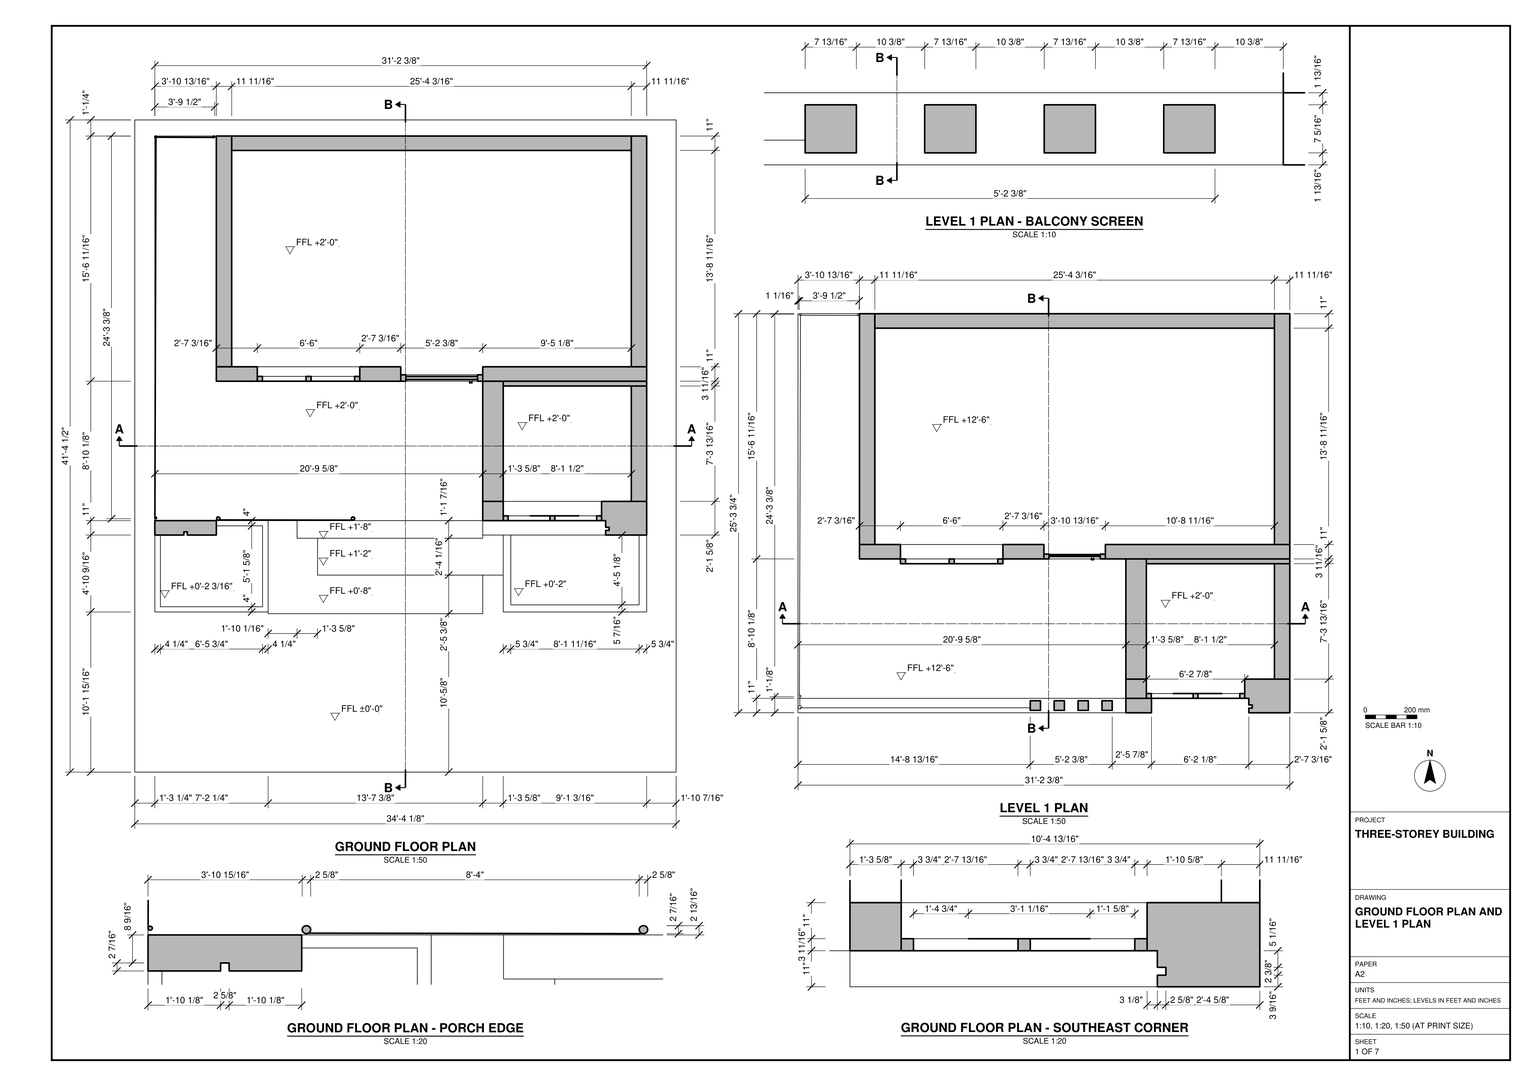
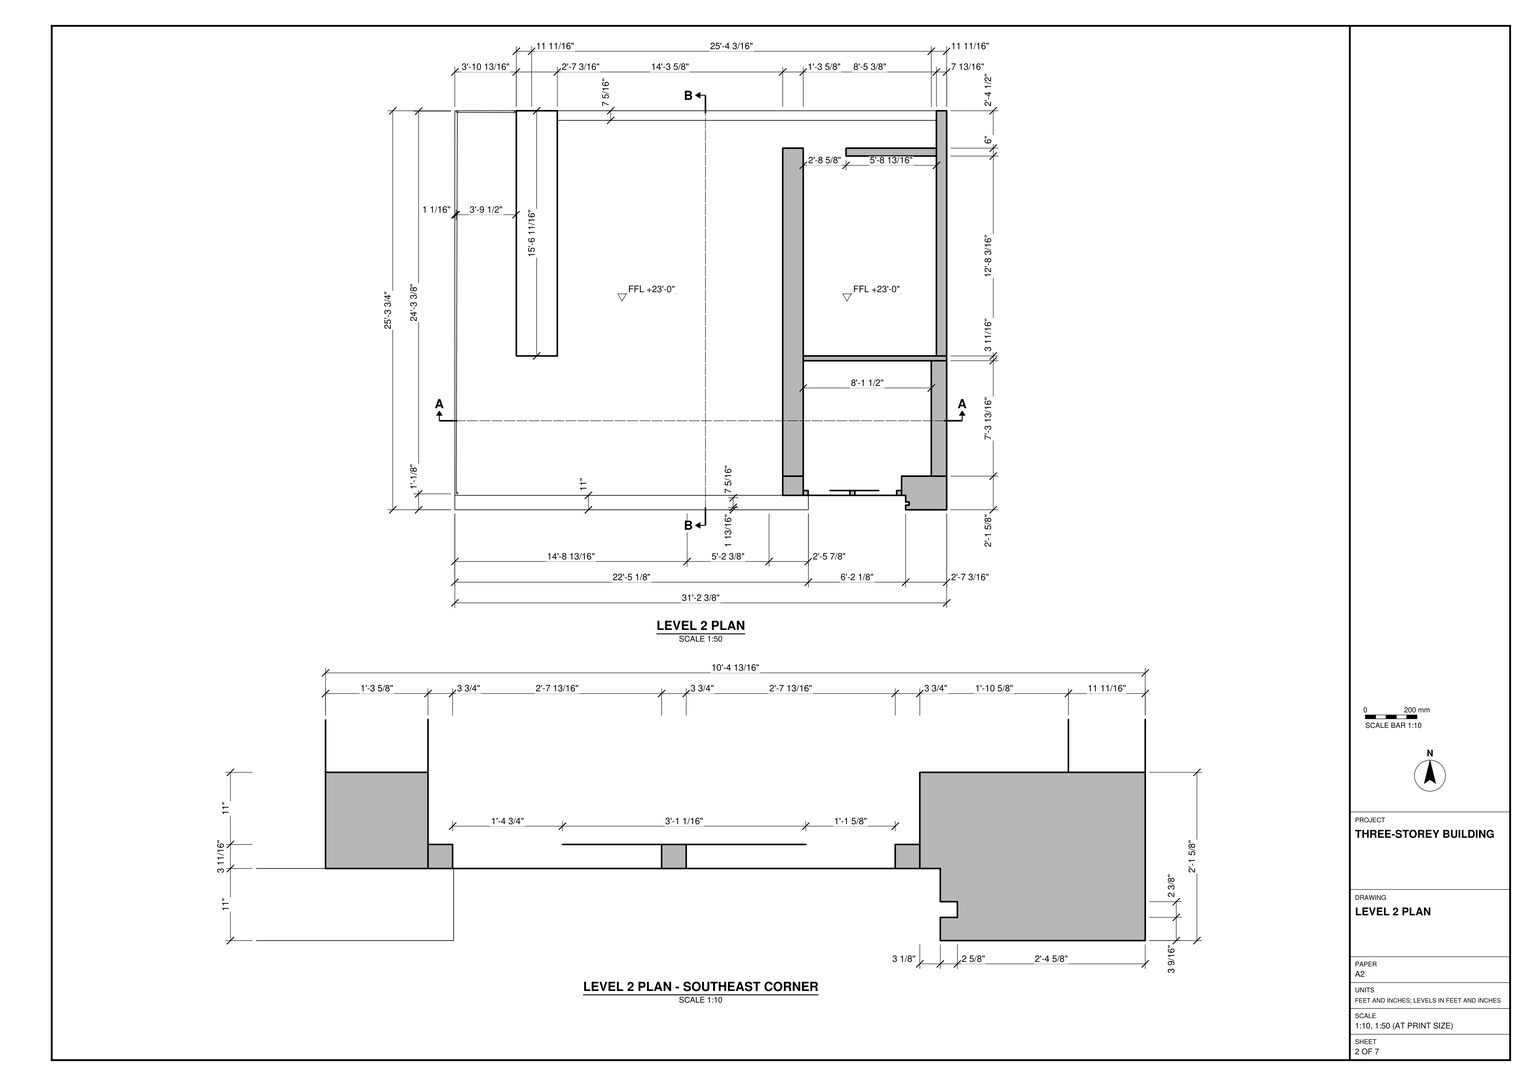
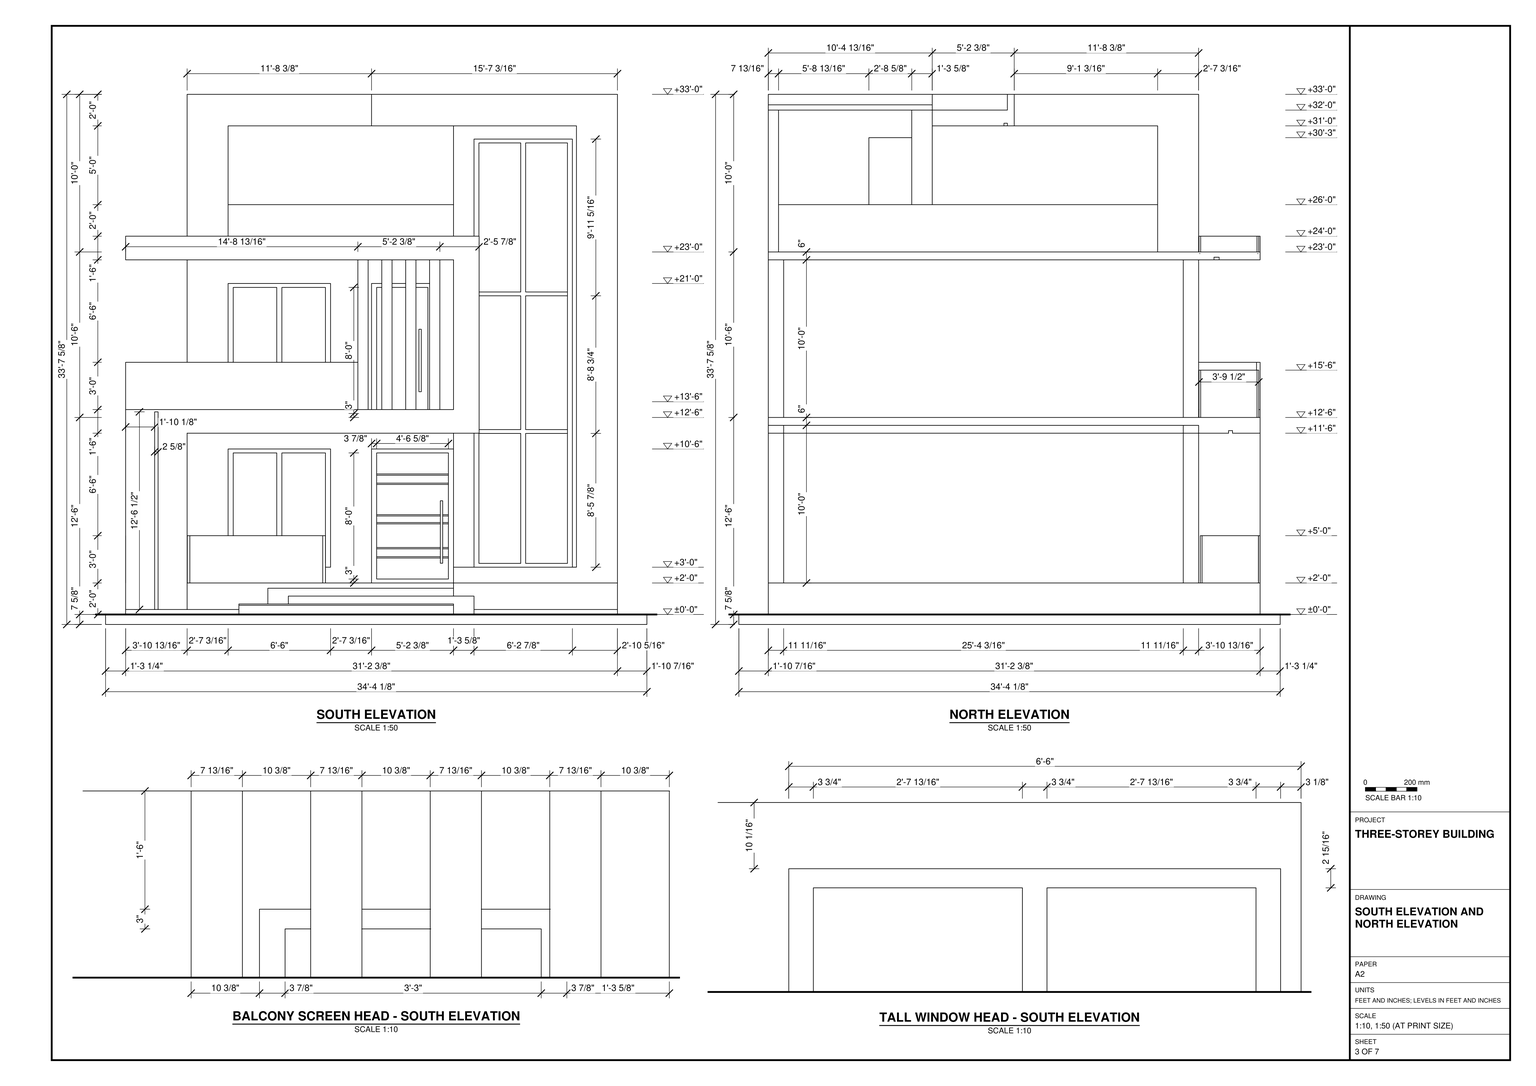
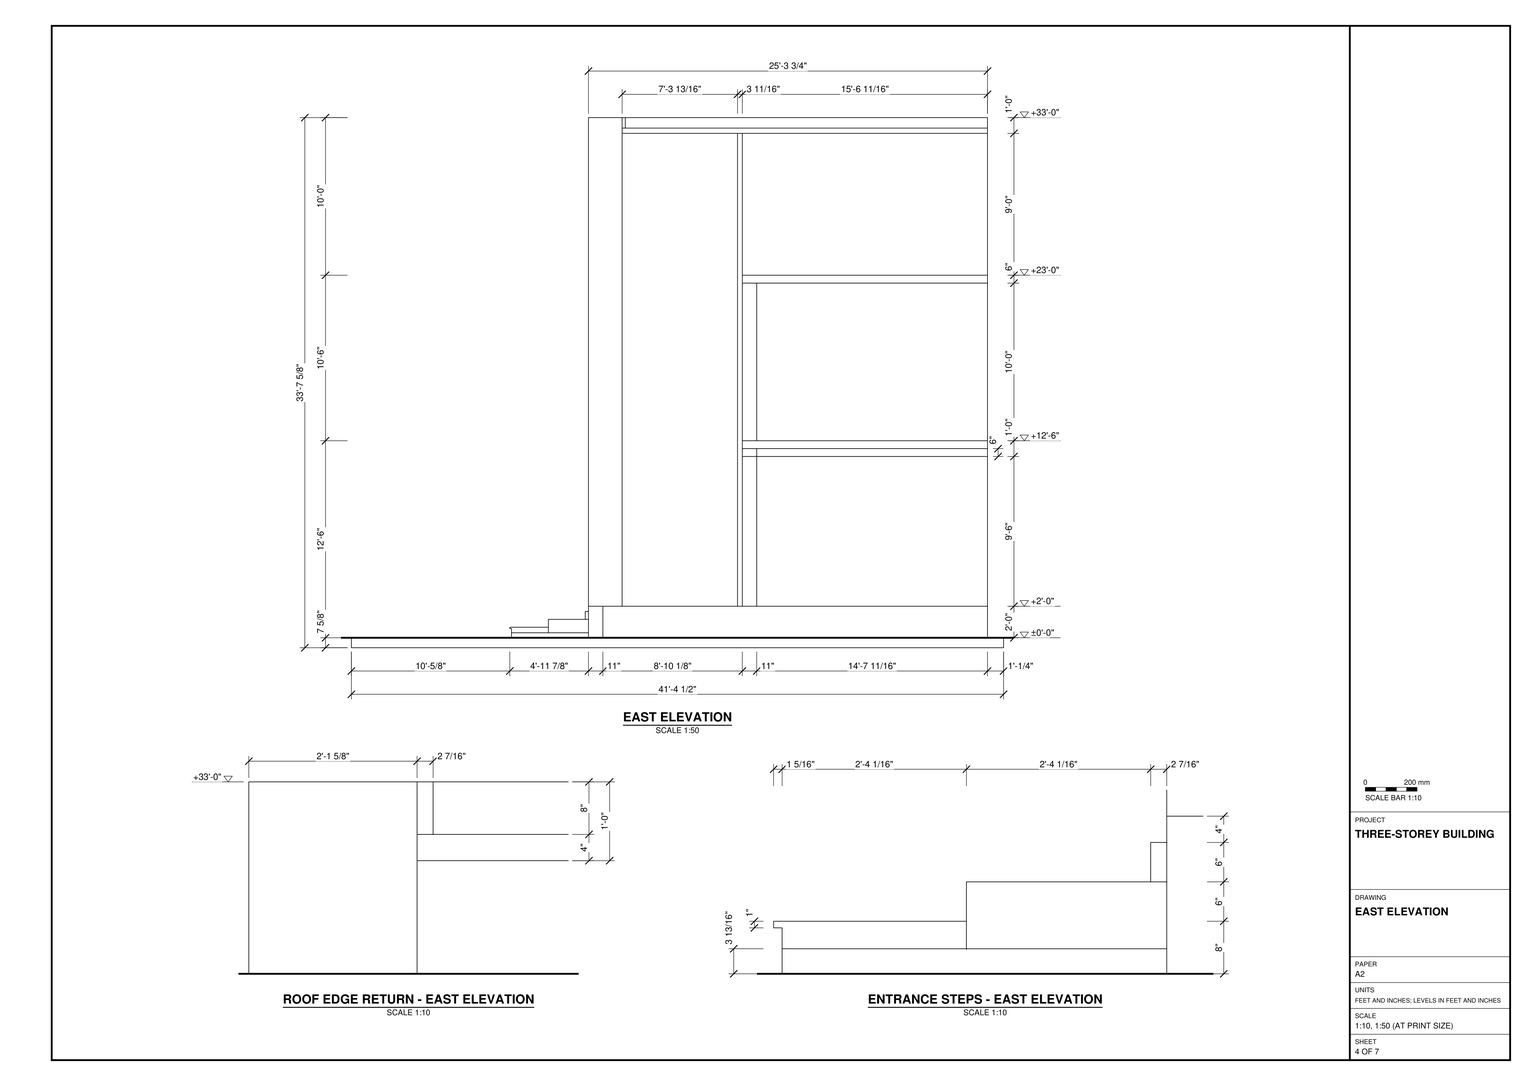
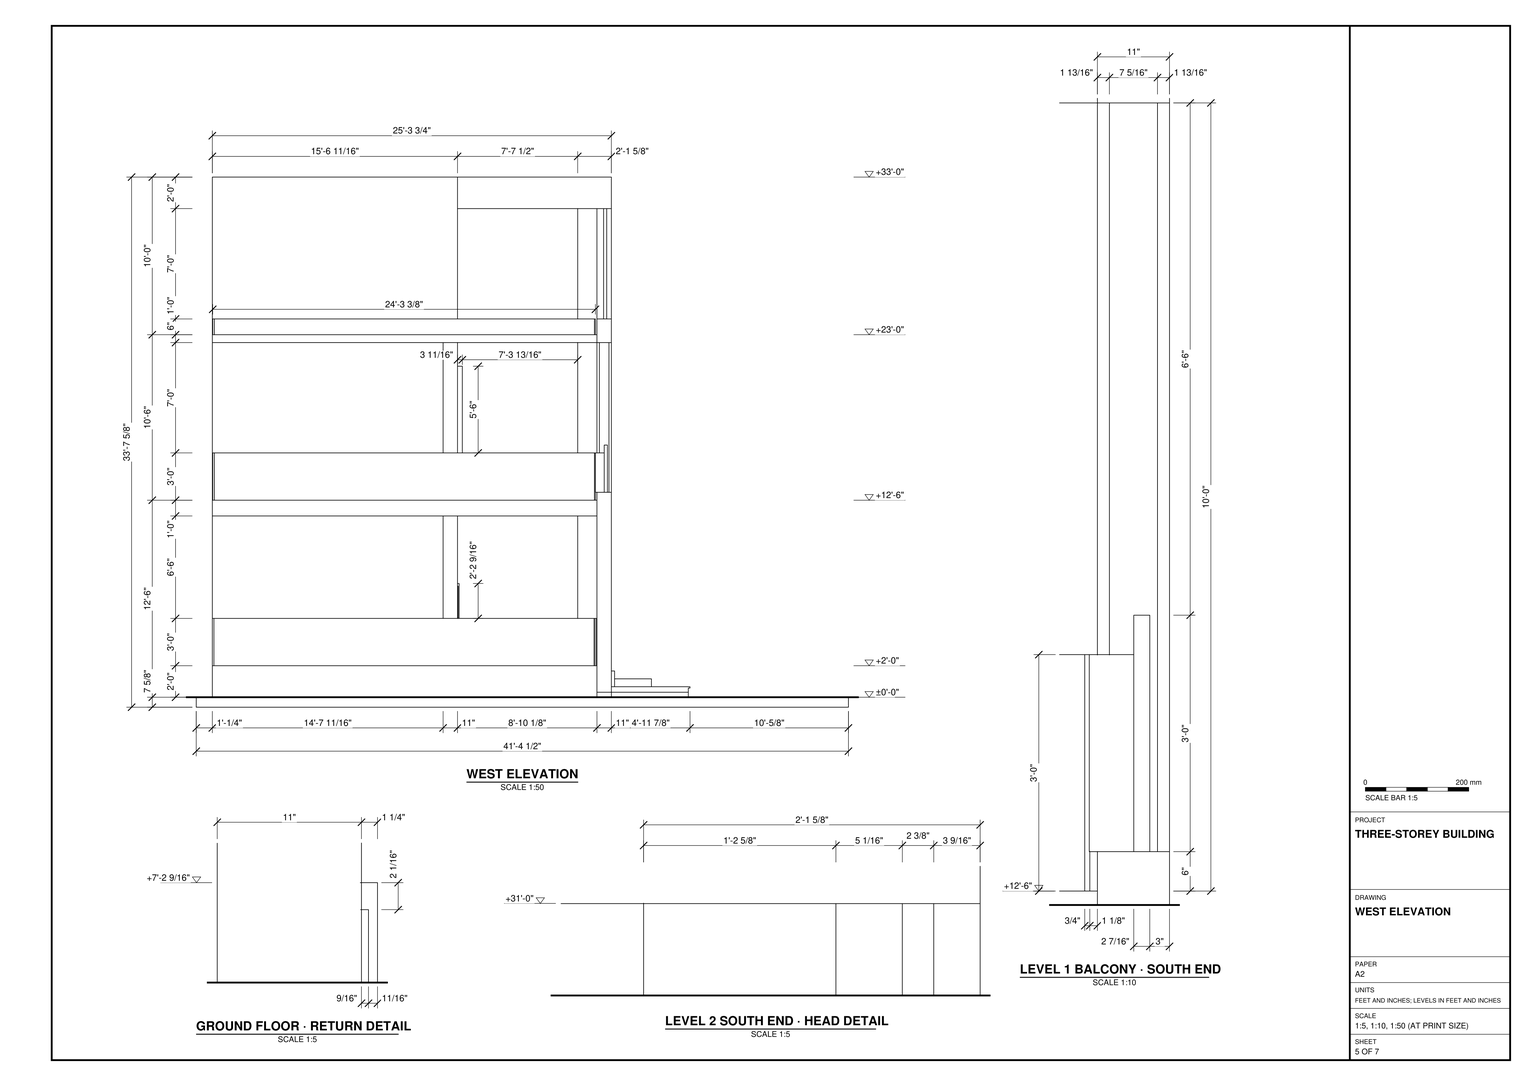
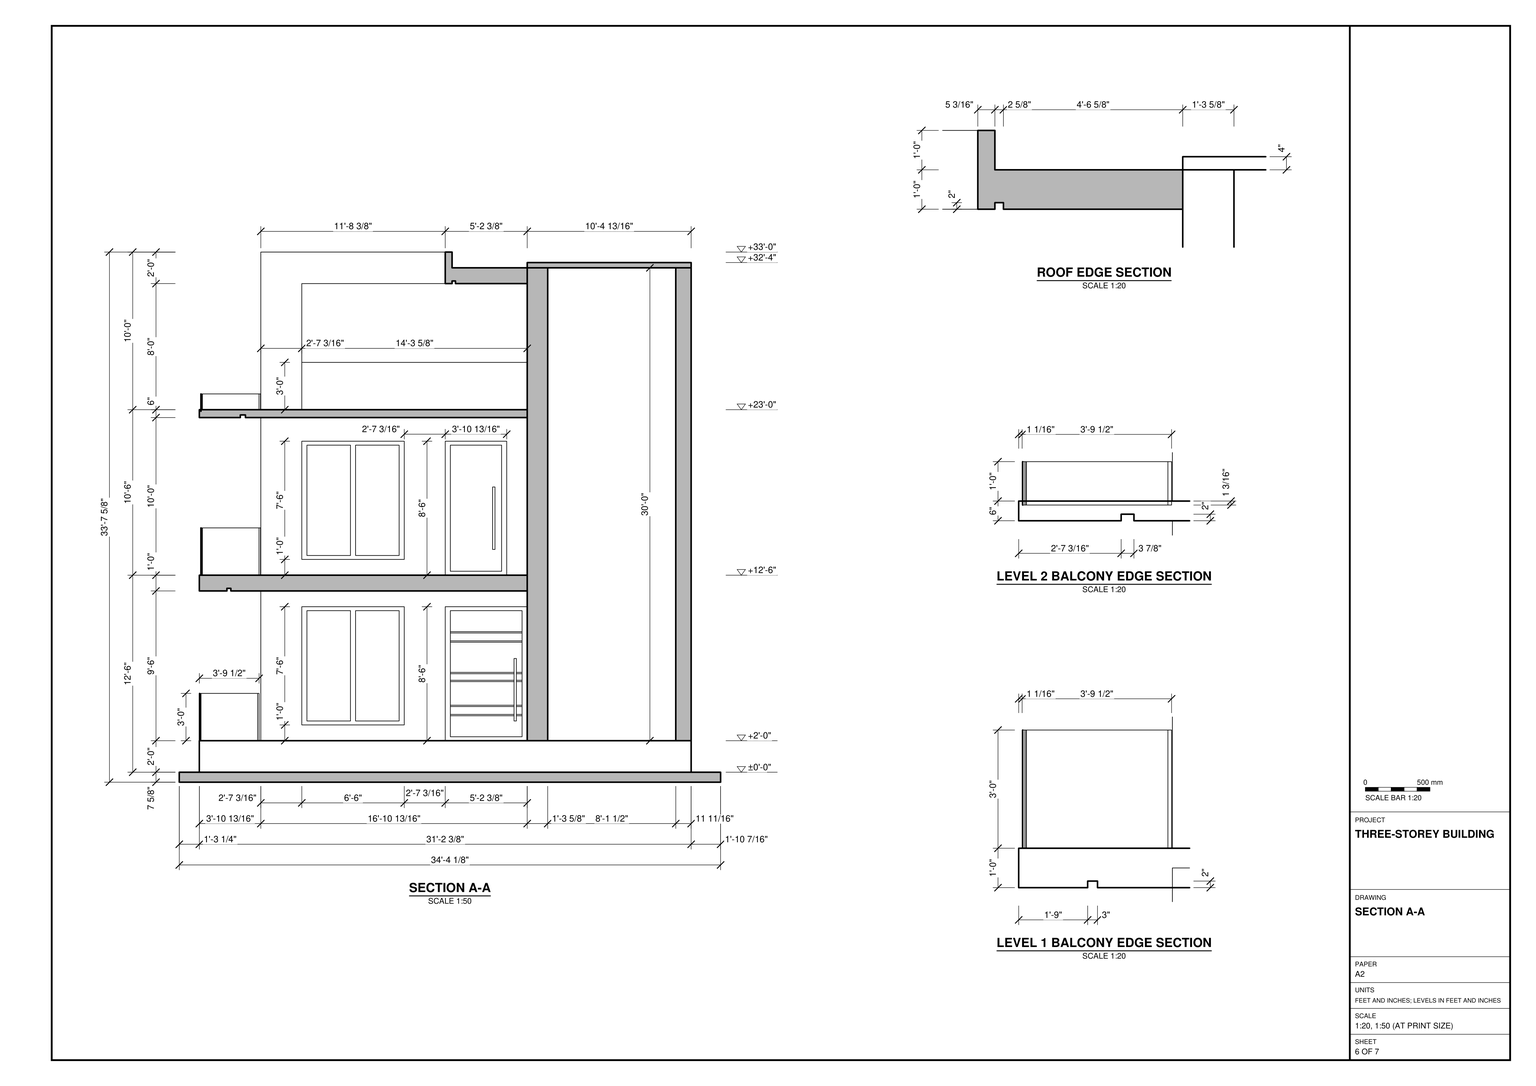
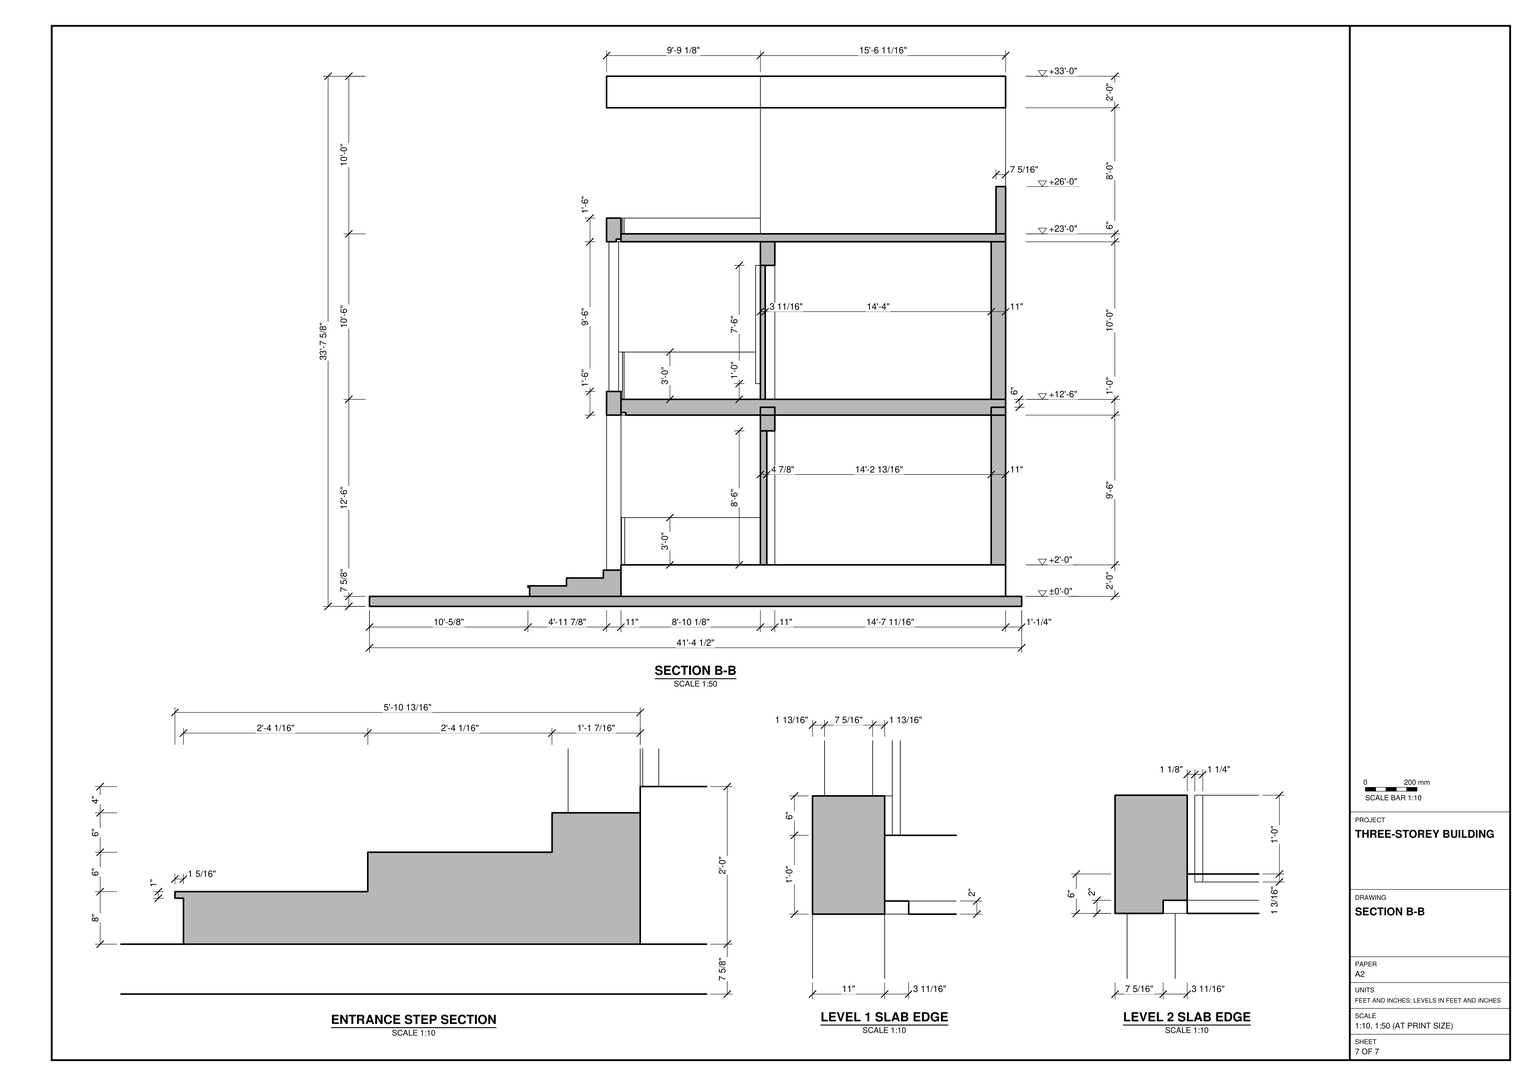
Build the three-storey building shown in task_files/diagram_01.pdf. Work in feet and inches. Including the base slab, the model must measure 34'-4 1/8" east to west, 41'-4 1/2" north to south and 33'-7 5/8" from bottom to top. Use ±0'-0" as the ground datum, +12'-6" for Level 1 and +23'-0" for Level 2. Distinguish the raised entrance floor from the ground datum.

Lay out the broad rear enclosure, the south-facing porch and the narrower southeast bay from the plans. Model the entrance steps, porch edge, walls at their drawn thicknesses, door and window openings, and projecting floor slabs. Align the Level 1 balcony with the porch below. Follow the enlarged details for the spacing of the balcony screen and the subdivisions of the tall southeast window. At Level 2, use the plan and elevations together to distinguish solid wall panels from open areas beneath the roof frame.

Keep walls, slabs, roof elements and each furniture or joinery piece shown in separate groups or components, and use components for repeated parts. Any decor or loose items shown may be represented by suitable library components. Save one SketchUp model as output_files/three_storey_building_with_a_screened_balcony.skp.

# SketchUp Ruby script. Lengths in inches.
U = 1.inch
M = Sketchup.active_model
def pt(a) = Geom::Point3d.new(a.map { |v| v * U })
def face(e, loops, mat)
  f = e.add_face(loops[0].map { |a| pt(a) })
  loops[1..].each { |l| e.add_face(l.map { |a| pt(a) }).erase! }
  f.material = f.back_material = mat if mat
  f
end
# faces: each face lists its corners as indices into pts; further lists are holes
def faces(e, pts, list, mat = nil) = list.each { |f| face(e, (f[0].is_a?(Array) ? f : [f]).map { |l| l.map { |i| pts[i] } }, mat) }
# xy, xz, yz: faces in a plane at the given z, y or x. An outline is a flat list of corners, or four numbers for a rectangle; further outlines are holes
def ring(l) = l.size == 4 ? [[l[0], l[1]], [l[2], l[1]], [l[2], l[3]], [l[0], l[3]]] : l.each_slice(2).to_a
def flat(e, list, mat, &to3) = list.each { |f| face(e, (f[0].is_a?(Array) ? f : [f]).map { |l| ring(l).map { |u, v| to3.(u, v) } }, mat) }
def xy(e, z, list, mat = nil) = flat(e, list, mat) { |x, y| [x, y, z] }
def xz(e, y, list, mat = nil) = flat(e, list, mat) { |x, z| [x, y, z] }
def yz(e, x, list, mat = nil) = flat(e, list, mat) { |y, z| [x, y, z] }
def lines(e, pts, list) = list.each { |a, b| e.add_line(pt(pts[a]), pt(pts[b])) }
# prism: a flat outline (further loops are holes) pulled along v
def prism(e, loops, v, mat = nil)
  f = face(e, loops, mat); d = Geom::Vector3d.new(v.map { |x| x * U })
  f.pushpull(f.normal.samedirection?(d) ? d.length : -d.length)
end
def box(e, o, s, mat = nil) = prism(e, [[o, [o[0] + s[0], o[1], o[2]], [o[0] + s[0], o[1] + s[1], o[2]], [o[0], o[1] + s[1], o[2]]]], [0, 0, s[2]], mat)
def at(x, y, z, deg = 0) = Geom::Transformation.translation(pt([x, y, z])) * Geom::Transformation.rotation(ORIGIN, Z_AXIS, deg.degrees)
def axes(o, x, y, z) = Geom::Transformation.new([*x, 0, *y, 0, *z, 0, *pt(o).to_a, 1])
def part(name) = M.definitions.add(name)
# library, detail: a bought-in or finely detailed component or shape, given as its bounding box
def library(name, o, s) = part(name).tap { |d| box(d.entities, o, s) }
def detail(e, o, s) = box(e.add_group.entities, o, s)
def put(e, d, t, mat = nil) = e.add_instance(d, t).tap { |i| i.material = mat if mat }
def group(e, t, mat = nil) = e.add_group.tap { |g| g.transformation = t; g.material = mat if mat }.entities
root = M.entities
M.materials.add("[Blinds Vertical Pattern]").color = [252, 252, 255]
M.materials.add("[Color G08]").color = [0, 102, 0]
M.materials.add("[Color M00]").color = [255, 255, 255]
M.materials.add("[Color M03]").color = [170, 170, 170]
M.materials.add("[Color M09]").color = [0, 0, 0]
M.materials.add("[Grass Dark Green]").color = [106, 157, 55]
M.materials.add("[Marble Carrara Floor Tile]").color = [204, 208, 219]
M.materials.add("[Marble Carrara Gold Floor Tile]").color = [225, 223, 217]
M.materials.add("[Metal Corrugated Shiny]").color = [193, 193, 193]
M.materials.add("[Metal Seamed]").color = [118, 119, 115]
M.materials.add("[Tile Mosaic Multi]").color = [160, 122, 114]
M.materials.add("[Translucent Glass Gray]").color = [255, 255, 255]
M.materials["[Translucent Glass Gray]"].alpha = 0.5
M.materials.add("[Translucent Glass Tinted]").color = [8, 201, 241]
M.materials["[Translucent Glass Tinted]"].alpha = 0.14
M.materials.add("[Wood Cherry Original]").color = [152, 86, 42]
M.materials.add("[Wood Veneer 02]").color = [190, 128, 91]
c1 = part("Group\#7")
xz(c1.entities,0,[[3,3,28.5,87],[31.5,3,57,87]],"[Translucent Glass Tinted]")
g1 = group(c1.entities,at(0,0,0),"[Color M09]")
prism(g1,[[[0,0,90],[0,0,0],[60,0,0],[60,0,90]],[[28.5,0,87],[28.5,0,3],[3,0,3],[3,0,87]],[[31.5,0,87],[57,0,87],[57,0,3],[31.5,0,3]]],[0,3,0])
c2 = part("Group\#8")
prism(c2.entities,[[[1.375,2,45.51],[1.375,2,47.5625],[1.375,0,47.5625],[1.375,0,0],[1.375,2,0],[1.375,2,1.44],[1.375,0.5625,1.44],[1.375,0.5625,45.51]]],[-1.375,0,0])
c3 = part("Group\#35")
prism(c3.entities,[[[1.26,1.97,0],[1.5,1.87,0],[1.71,1.71,0],[1.87,1.5,0],[1.97,1.26,0],[2,1,0],[1.97,0.74,0],[1.87,0.5,0],[1.71,0.29,0],[1.5,0.13,0],[1.26,0.03,0],[1,0,0],[0.74,0.03,0],[0.5,0.13,0],[0.29,0.29,0],[0.13,0.5,0],[0.03,0.74,0],[0,1,0],[0.03,1.26,0],[0.13,1.5,0],[0.29,1.71,0],[0.5,1.87,0],[0.74,1.97,0],[1,2,0]]],[0,0,36])
c4 = part("Group\#34")
prism(c4.entities,[[[0.5,0,0],[0.37,0.02,0],[0.25,0.07,0],[0.15,0.15,0],[0.07,0.25,0],[0.02,0.37,0],[0,0.5,0],[0.02,0.63,0],[0.07,0.75,0],[0.15,0.85,0],[0.25,0.93,0],[0.37,0.98,0],[0.5,1,0],[0.63,0.98,0],[0.75,0.93,0],[0.85,0.85,0],[0.93,0.75,0],[0.98,0.63,0],[1,0.5,0],[0.98,0.37,0],[0.93,0.25,0],[0.85,0.15,0],[0.75,0.07,0],[0.63,0.02,0]]],[0,0,36])
c5 = part("Group\#44")
p = [[0.82,237.83,36],[0.02,0.63,36],[0.02,0.63,0],[0.82,237.83,0],[44.39,237.96,0],[44.39,237.96,36],
  [1.21,238.0625,36],[1.21,238.0625,0]]
faces(c5.entities,p,[[0,1,2,3],[4,5,6,7]],"[Translucent Glass Gray]")
put(c5.entities,c4,axes([44.2,237.8125,0],[1.3,0,0],[0,1,0],[0,0,1]))
put(c5.entities,c4,axes([0,237.8125,0],[1.3,0,0],[0,1,0],[0,0,1]))
put(c5.entities,c4,axes([0,0,0],[1.3,0,0],[0,1,0],[0,0,1]))
prism(root,[[[313.09,449.78,269.85],[381.88,449.78,269.85],[381.88,449.78,377.85],[280.48,449.78,377.85],[280.48,449.78,356.87],[313.09,449.78,356.87]]],[0,6,0])
xy(root,17.85,[[377.98,206.09,389.68,293.93]])
xy(root,377.85,[[377.98,206.09,389.68,293.93]])
xz(root,206.09,[[377.98,17.85,389.68,377.85]])
xz(root,293.93,[[377.98,17.85,389.68,377.85]])
yz(root,377.98,[[206.09,17.85,293.93,377.85]])
p = [[64.16,191.99,53.85],[165.32,191.83,53.85],[165.32,191.83,17.85],[64.16,191.99,17.85],[16.66,192.6875,179.85],[16.64,185.91,179.85],
  [16.64,185.91,149.85],[16.66,192.6875,149.85],[264.88,137.77,-0.15],[101.5,137.77,-0.15],[264.88,137.77,0.85],[101.5,137.77,0.85]]
faces(root,p,[[0,1,2,3],[4,5,6,7]],"[Translucent Glass Gray]")
lines(root,p,[[8,9],[10,11]])
g2 = group(root,at(62.08,191.45,-6.15),"[Marble Carrara Floor Tile]")
box(g2,[-46.8,0,0],[374.4,292.8,24])
g3 = group(root,at(73.78,297.59,17.85),"[Color M03]")
prism(g3,[[[315.9,10.98,0],[191.1,10.98,0],[191.1,10.98,102],[128.7,10.98,102],[128.7,10.98,0],[-11.7,10.98,0],[-11.7,10.98,120],[315.9,10.98,120]],[[97.5,10.98,12],[97.5,10.98,102],[19.5,10.98,102],[19.5,10.98,12]]],[0,-10.98,0])
g4 = group(root,at(202.48,296.37,17.85))
g5 = group(g4,at(0,2.44,0),"[Wood Cherry Original]")
prism(g5,[[[0,3.66,0],[0,3.66,102],[62.4,3.66,102],[62.4,3.66,0]],[[3.9,3.66,99],[3.9,3.66,3],[58.5,3.66,3],[58.5,3.66,99]]],[0,-4.88,0])
g6 = group(g4,at(3.9,2.44,3),"[Wood Cherry Original]")
xy(g6,0,[[0,0,54.6,2.44]])
xy(g6,16,[[0,0,54.6,0.61]])
xy(g6,17,[[0,0,54.6,0.61]])
xy(g6,23,[[0,0,54.6,0.61]])
xy(g6,24,[[0,0,54.6,0.61]])
xy(g6,42,[[0,0,54.6,0.61]])
xy(g6,43,[[0,0,54.6,0.61]])
xy(g6,48,[[0,0,54.6,0.61]])
xy(g6,49,[[0,0,54.6,0.61]])
xy(g6,72,[[0,0,54.6,0.61]])
xy(g6,73,[[0,0,54.6,0.61]])
xy(g6,79,[[0,0,54.6,0.61]])
xy(g6,80,[[0,0,54.6,0.61]])
xy(g6,96,[[0,0,54.6,2.44]])
xz(g6,0,[[0,0,54.6,16],[0,17,54.6,23],[0,43,54.6,48],[0,49,54.6,72],[0,73,54.6,79],
  [0,80,54.6,96]])
xz(g6,0,[[0,24,54.6,42]],"[Wood Cherry Original]")
xz(g6,0.61,[[0,16,54.6,17],[0,23,54.6,24],[0,42,54.6,43],[0,48,54.6,49],[0,72,54.6,73],
  [0,79,54.6,80]])
xz(g6,2.44,[[0,0,54.6,96]])
yz(g6,0,[[0,0,0,16,0.61,16,0.61,17,0,17,0,23,0.61,23,0.61,24,0,24,0,42,0.61,42,0.61,43,0,43,0,48,0.61,48,0.61,49,0,49,0,72,0.61,72,0.61,73,0,73,0,79,0.61,79,0.61,80,0,80,0,96,2.44,96,2.44,0]])
yz(g6,54.6,[[0,0,2.44,0,2.44,96,0,96,0,80,0.61,80,0.61,79,0,79,0,73,0.61,73,0.61,72,0,72,0,49,0.61,49,0.61,48,0,48,0,43,0.61,43,0.61,42,0,42,0,24,0.61,24,0.61,23,0,23,0,17,0.61,17,0.61,16,0,16]])
put(root,c1,axes([93.28,297.59,29.85],[1.3,0,0],[0,1.22,0],[0,0,1]))
put(root,c2,axes([254.84,296.37,32.88],[1.3,0,0],[0,1.22,0],[0,0,1]),"[Metal Seamed]")
g7 = group(root,at(62.08,308.57,17.85))
box(g7,[0,0,0],[11.7,175.68,120])
g8 = group(root,at(73.78,473.27,17.85))
box(g8,[0,0,0],[304.2,10.98,120])
g9 = group(root,at(377.98,308.57,17.85))
box(g9,[0,0,0],[11.7,175.68,120])
g10 = group(root,at(62.08,297.59,137.85))
xy(g10,-6,[[-46.8,-106.14,-25.8,186.66],[-22.8,-102.48,-22.8,186.66,327.6,186.66,327.6,0,202.8,0,202.8,-102.48]])
xy(g10,-4,[[-25.8,-106.14,202.8,-102.48],[-25.8,-102.48,-22.8,186.66]],"[Color M09]")
xy(g10,6,[[-46.8,-106.14,202.8,-106.14,202.8,0,327.6,0,327.6,186.66,-46.8,186.66]])
xz(g10,-106.14,[[-46.8,-6,-25.8,-6,-25.8,-4,202.8,-4,202.8,6,-46.8,6]])
xz(g10,-102.48,[[-22.8,-6,202.8,-4]],"[Color M09]")
xz(g10,0,[[202.8,-6,327.6,6]])
xz(g10,186.66,[[-46.8,-6,-46.8,6,327.6,6,327.6,-6,-22.8,-6,-22.8,-4,-25.8,-4,-25.8,-6]])
yz(g10,-46.8,[[-106.14,-6,186.66,6]])
yz(g10,-25.8,[[-106.14,-6,-102.48,-4],[-102.48,-6,186.66,-4]],"[Color M09]")
yz(g10,-22.8,[[-102.48,-6,186.66,-4]],"[Color M09]")
yz(g10,202.8,[[-102.48,-6,0,-6,0,6,-106.14,6,-106.14,-4,-102.48,-4]])
yz(g10,327.6,[[0,-6,186.66,6]])
g11 = group(root,at(62.08,297.59,143.85),"[Color M03]")
prism(g11,[[[140.4,10.98,0],[0,10.98,0],[0,10.98,120],[327.6,10.98,120],[327.6,10.98,0],[187.2,10.98,0],[187.2,10.98,102],[140.4,10.98,102]],[[31.2,10.98,102],[31.2,10.98,12],[109.2,10.98,12],[109.2,10.98,102]]],[0,-10.98,0])
g12 = group(root,at(377.98,308.57,143.85))
box(g12,[0,0,0],[11.7,175.68,120])
g13 = group(root,at(73.78,473.27,143.85))
box(g13,[0,0,0],[304.2,10.98,120])
g14 = group(root,at(62.08,308.57,143.85))
box(g14,[0,0,0],[11.7,175.68,120])
put(root,c1,axes([93.28,293.93,155.85],[1.3,0,0],[0,1.22,0],[0,0,1]))
g15 = group(root,at(202.48,297.59,143.85),"[Wood Cherry Original]")
prism(g15,[[[46.8,3.66,0],[0,3.66,0],[0,3.66,102],[46.8,3.66,102]],[[42.9,3.66,99],[3.9,3.66,99],[3.9,3.66,3],[42.9,3.66,3]]],[0,-3.66,0])
g16 = group(root,at(206.38,299.42,146.85),"[Wood Cherry Original]")
box(g16,[0,0,0],[39,1.22,96])
put(root,c2,axes([238.55,296.98,163.44],[1.3,0,0],[0,1.22,0],[0,0,1]),"[Metal Seamed]")
g17 = group(root,at(62.08,297.59,263.85))
xy(g17,0,[[-46.8,-106.14,-15.6,186.66],[-11.7,-106.14,-11.7,186.66,327.6,186.66,327.6,0,202.8,0,202.8,-106.14]])
xy(g17,2,[[-15.6,-106.14,-11.7,186.66]],"[Color M09]")
xy(g17,6,[[-46.8,-106.14,202.8,-106.14,202.8,0,327.6,0,327.6,186.66,-46.8,186.66]])
xz(g17,-106.14,[[-46.8,0,-15.6,0,-15.6,2,-11.7,2,-11.7,0,202.8,0,202.8,6,-46.8,6]],"[Color M09]")
xz(g17,0,[[202.8,0,327.6,6]])
xz(g17,186.66,[[-46.8,0,-46.8,6,327.6,6,327.6,0,-11.7,0,-11.7,2,-15.6,2,-15.6,0]])
yz(g17,-46.8,[[-106.14,0,186.66,6]])
yz(g17,-15.6,[[-106.14,0,186.66,2]],"[Color M09]")
yz(g17,-11.7,[[-106.14,0,186.66,2]],"[Color M09]")
yz(g17,202.8,[[-106.14,0,0,6]])
yz(g17,327.6,[[0,0,186.66,6]])
g18 = group(root,at(264.88,206.09,17.85),"[Color M09]")
xy(g18,0,[[0,0,15.6,91.5]])
xy(g18,252,[[0,91.5,15.6,249.6875]])
xy(g18,360,[[0,0,15.6,249.6875]],"[Color M00]")
xz(g18,0,[[0,0,15.6,360]])
xz(g18,91.5,[[0,0,15.6,252]])
xz(g18,249.6875,[[0,252,15.6,360]],"[Color M00]")
yz(g18,0,[[0,0,91.5,252]])
yz(g18,0,[[0,252,249.6875,360]],"[Color M00]")
yz(g18,15.6,[[0,0,91.5,0,91.5,252,249.6875,252,249.6875,360,0,360]],"[Color M00]")
g19 = group(root,at(264.88,191.45,17.85))
xy(g19,0,[[0,-10.98,124.8,14.64]])
xy(g19,12,[[0,-10.98,93.6,-10.98,93.6,-7.45,96.2,-7.45,96.2,-5.05,93.6,-5.05,93.6,14.64,15.6,14.64,15.6,0,0,0]],"[Color M09]")
xy(g19,12.04,[[90.48,0,93.6,14.64]])
xy(g19,337.92,[[15.6,0,90.48,14.64]])
xy(g19,348,[[-62.4,-10.98,-62.4,292.8,-57.2,292.8,-57.2,-7.45,93.6,-7.45,93.6,-10.98],[[-54.6,-5.05,-54.6,292.8,0,292.8,0,0,93.6,0,93.6,-5.05],[-49.4,30.5,-7.8,45.14],[-49.4,118.34,-7.8,132.98],[-49.4,1.22,-7.8,15.86],[-49.4,147.62,-7.8,162.26],[-49.4,59.78,-7.8,74.42],[-49.4,215.94,-7.8,230.58],[-49.4,196.42,-7.8,211.06],[-49.4,176.9,-7.8,191.54],[-49.4,274.5,-7.8,289.14],[-49.4,245.22,-7.8,259.86],[-49.4,89.06,-7.8,103.7]]])
xy(g19,348,[[93.6,-7.45,96.2,-5.05]],"[Color M09]")
xy(g19,350,[[-57.2,-7.45,93.6,-5.05],[-57.2,-5.05,-54.6,292.8]],"[Color M09]")
xy(g19,360,[[[-57.2,17.08,0,292.8],[-49.4,30.5,-7.8,45.14],[-49.4,118.34,-7.8,132.98],[-49.4,59.78,-7.8,74.42],[-49.4,147.62,-7.8,162.26],[-49.4,176.9,-7.8,191.54],[-49.4,196.42,-7.8,211.06],[-49.4,215.94,-7.8,230.58],[-49.4,245.22,-7.8,259.86],[-49.4,274.5,-7.8,289.14],[-49.4,89.06,-7.8,103.7]]])
xy(g19,372,[[[-62.4,-10.98,124.8,-10.98,124.8,14.64,0,14.64,0,17.08,-57.2,17.08,-57.2,14.64,-62.4,14.64],[-49.4,1.22,-7.8,15.86]],[-62.4,14.64,-57.2,292.8]])
xz(g19,-10.98,[[0,0,124.8,0,124.8,372,-62.4,372,-62.4,348,93.6,348,93.6,12,0,12]])
xz(g19,-7.45,[[93.6,12,96.2,348],[-57.2,348,93.6,350]],"[Color M09]")
xz(g19,-5.05,[[93.6,12,96.2,348],[-54.6,348,93.6,350]],"[Color M09]")
xz(g19,0,[[0,12,15.6,12,15.6,337.92,90.48,337.92,90.48,12.04,93.6,12.04,93.6,348,0,348]],"[Color M09]")
xz(g19,1.22,[[-49.4,348,-7.8,372]])
xz(g19,14.64,[[[0,0,124.8,372],[15.6,12,93.6,12,93.6,12.04,90.48,12.04,90.48,337.92,15.6,337.92]]])
xz(g19,15.86,[[-49.4,348,-7.8,372]])
xz(g19,17.08,[[-57.2,360,0,372]])
xz(g19,30.5,[[-49.4,348,-7.8,360]])
xz(g19,45.14,[[-49.4,348,-7.8,360]])
xz(g19,59.78,[[-49.4,348,-7.8,360]])
xz(g19,74.42,[[-49.4,348,-7.8,360]])
xz(g19,89.06,[[-49.4,348,-7.8,360]])
xz(g19,103.7,[[-49.4,348,-7.8,360]])
xz(g19,118.34,[[-49.4,348,-7.8,360]])
xz(g19,132.98,[[-49.4,348,-7.8,360]])
xz(g19,147.62,[[-49.4,348,-7.8,360]])
xz(g19,162.26,[[-49.4,348,-7.8,360]])
xz(g19,176.9,[[-49.4,348,-7.8,360]])
xz(g19,191.54,[[-49.4,348,-7.8,360]])
xz(g19,196.42,[[-49.4,348,-7.8,360]])
xz(g19,211.06,[[-49.4,348,-7.8,360]])
xz(g19,215.94,[[-49.4,348,-7.8,360]])
xz(g19,230.58,[[-49.4,348,-7.8,360]])
xz(g19,245.22,[[-49.4,348,-7.8,360]])
xz(g19,259.86,[[-49.4,348,-7.8,360]])
xz(g19,274.5,[[-49.4,348,-7.8,360]])
xz(g19,289.14,[[-49.4,348,-7.8,360]])
xz(g19,292.8,[[-62.4,348,-62.4,372,-57.2,372,-57.2,360,0,360,0,348,-54.6,348,-54.6,350,-57.2,350,-57.2,348]])
yz(g19,-62.4,[[-10.98,348,292.8,372]])
yz(g19,-57.2,[[-7.45,348,-5.05,350],[17.08,360,292.8,372]])
yz(g19,-57.2,[[-5.05,348,292.8,350]],"[Color M09]")
yz(g19,-54.6,[[-5.05,348,292.8,350]],"[Color M09]")
yz(g19,-49.4,[[1.22,348,15.86,372],[30.5,348,45.14,360],[59.78,348,74.42,360],[89.06,348,103.7,360],[118.34,348,132.98,360],
  [147.62,348,162.26,360],[176.9,348,191.54,360],[196.42,348,211.06,360],[215.94,348,230.58,360],[245.22,348,259.86,360],
  [274.5,348,289.14,360]])
yz(g19,-7.8,[[1.22,348,6.1,372],[6.1,348,15.86,372],[30.5,348,35.38,360],[35.38,348,45.14,360],[59.78,348,64.66,360],
  [64.66,348,74.42,360],[89.06,348,93.94,360],[93.94,348,103.7,360],[118.34,348,123.22,360],[123.22,348,132.98,360],
  [147.62,348,152.5,360],[152.5,348,162.26,360],[176.9,348,186.66,360],[186.66,348,191.54,360],[196.42,348,206.18,360],
  [206.18,348,211.06,360],[215.94,348,220.82,360],[220.82,348,230.58,360],[245.22,348,259.86,360],[274.5,348,289.14,360]])
yz(g19,0,[[-10.98,0,-10.98,12,0,12,0,348,14.64,348,14.64,0],[14.64,348,292.8,360],[14.64,360,17.08,372]])
yz(g19,15.6,[[0,12,14.64,337.92]])
yz(g19,90.48,[[0,12.04,14.64,337.92]])
yz(g19,93.6,[[-10.98,12,-7.45,348],[-5.05,12,-5.05,348,0,348,0,12.04,14.64,12.04,14.64,12]])
yz(g19,93.6,[[-7.45,348,-5.05,350]],"[Color M09]")
yz(g19,96.2,[[-7.45,12,-5.05,348]],"[Color M09]")
yz(g19,124.8,[[-10.98,0,14.64,372]])
g20 = group(root,at(280.48,191.45,29.85),"[Blinds Vertical Pattern]")
xz(g20,0,[[3.74,2.91,35.57,101.85],[39.3125,2.91,71.14,101.85],[3.74,104.76,35.57,206.61],[39.3125,104.76,71.14,206.61],[3.74,209.52,35.57,323.01],
  [39.3125,209.52,71.14,323.01]],"[Translucent Glass Tinted]")
g21 = group(g20,at(0,0,0),"[Color M09]")
xy(g21,0,[[0,0,74.88,3.66]])
xy(g21,2.91,[[3.74,0,35.57,3.66],[39.3125,0,71.14,3.66]])
xy(g21,101.85,[[3.74,0,35.57,3.66],[39.3125,0,71.14,3.66]])
xy(g21,104.76,[[3.74,0,35.57,3.66],[39.3125,0,71.14,3.66]])
xy(g21,206.61,[[3.74,0,35.57,3.66],[39.3125,0,71.14,3.66]])
xy(g21,209.52,[[3.74,0,35.57,3.66],[39.3125,0,71.14,3.66]])
xy(g21,323.01,[[3.74,0,35.57,3.66],[39.3125,0,71.14,3.66]])
xy(g21,325.92,[[0,0,74.88,3.66]])
xz(g21,0,[[[0,0,74.88,325.92],[39.3125,2.91,39.3125,101.85,71.14,101.85,71.14,104.76,39.3125,104.76,39.3125,206.61,71.14,206.61,71.14,209.52,39.3125,209.52,39.3125,323.01,71.14,323.01,71.14,2.91],[3.74,2.91,3.74,323.01,35.57,323.01,35.57,209.52,3.74,209.52,3.74,206.61,35.57,206.61,35.57,104.76,3.74,104.76,3.74,101.85,35.57,101.85,35.57,2.91]]])
xz(g21,3.66,[[[0,0,74.88,325.92],[39.3125,2.91,71.14,2.91,71.14,323.01,39.3125,323.01,39.3125,209.52,71.14,209.52,71.14,206.61,39.3125,206.61,39.3125,104.76,71.14,104.76,71.14,101.85,39.3125,101.85],[3.74,2.91,35.57,2.91,35.57,101.85,3.74,101.85,3.74,104.76,35.57,104.76,35.57,206.61,3.74,206.61,3.74,209.52,35.57,209.52,35.57,323.01,3.74,323.01]]])
yz(g21,0,[[0,0,3.66,325.92]])
yz(g21,3.74,[[0,2.91,3.66,101.85],[0,101.85,3.66,104.76],[0,104.76,3.66,206.61],[0,206.61,3.66,209.52],[0,209.52,3.66,323.01]])
yz(g21,35.57,[[0,2.91,3.66,101.85],[0,104.76,3.66,206.61],[0,209.52,3.66,323.01]])
yz(g21,39.3125,[[0,2.91,3.66,101.85],[0,104.76,3.66,206.61],[0,209.52,3.66,323.01]])
yz(g21,71.14,[[0,2.91,3.66,101.85],[0,101.85,3.66,104.76],[0,104.76,3.66,206.61],[0,206.61,3.66,209.52],[0,209.52,3.66,323.01]])
yz(g21,74.88,[[0,0,3.66,325.92]])
g22 = group(root,at(300.95,195.11,32.85))
xz(g22,0,[[0,0,37.05,330]],"[Blinds Vertical Pattern]")
g23 = group(root,at(101.5,120.61,-6.15),"[Marble Carrara Floor Tile]")
xy(g23,0,[[0,1.3,163.375,5.28],[0,5.28,163.375,70.84],[163.375,29.36,178.98,70.84]])
xy(g23,7,[[0,0,163.375,1.3]])
xy(g23,8,[[0,0,163.375,0,163.375,29.36,37.63,29.36,37.63,57.42,22.03,57.42,22.03,70.84,0,70.84]])
xy(g23,14,[[37.63,29.36,178.98,29.36,178.98,70.84,163.375,70.84,163.375,57.42,37.63,57.42]])
xy(g23,20,[[22.03,57.42,163.375,70.84]])
xz(g23,0,[[0,7,163.375,8]])
xz(g23,1.3,[[0,0,163.375,7]])
xz(g23,29.36,[[163.375,0,178.98,0,178.98,14,37.63,14,37.63,8,163.375,8]])
xz(g23,57.42,[[22.03,8,37.63,8,37.63,14,163.375,14,163.375,20,22.03,20]])
xz(g23,70.84,[[0,0,163.375,6],[163.375,0,163.375,6,0,6,0,8,22.03,8,22.03,20,163.375,20,163.375,14,178.98,14,178.98,0]])
yz(g23,0,[[1.3,0,1.3,7,0,7,0,8,70.84,8,70.84,0]])
yz(g23,22.03,[[57.42,8,70.84,20]])
yz(g23,37.63,[[29.36,8,57.42,14]])
yz(g23,163.375,[[1.3,0,29.36,0,29.36,8,0,8,0,7,1.3,7],[29.36,0,70.84,6],[57.42,14,70.84,20]])
yz(g23,178.98,[[29.36,0,70.84,14]])
g24 = group(root,at(264.88,180.47,-6.15),"[Marble Carrara Floor Tile]")
xy(g24,0,[[0,0,124.8,10.98]],"[Color M00]")
xy(g24,24,[[0,0,124.8,10.98]],"[Color M00]")
xz(g24,0,[[0,0,124.8,24]],"[Color M00]")
xz(g24,10.98,[[0,0,124.8,24]],"[Color M00]")
yz(g24,0,[[0,0,10.98,24]],"[Color M00]")
yz(g24,124.8,[[0,0,10.98,24]],"[Color M00]")
g25 = group(root,at(30.88,180.47,-6.15))
xy(g25,0,[[-15.6,0,-15.6,10.98,31.2,10.98,31.2,0,9.1,0,9.1,2.44,6.5,2.44,6.5,0]])
xy(g25,138,[[31.2,0,253.5,10.98]])
xy(g25,154.29,[[6.5,0,9.1,2.44]])
xy(g25,156,[[-15.6,0,234,10.98]])
xy(g25,270,[[-15.6,0,-15.6,10.98,15.6,10.98,15.6,7.32,234,7.32,234,0]])
xy(g25,272,[[15.6,7.32,234,10.98]],"[Color M09]")
xy(g25,288,[[-15.6,0,253.5,10.98]])
xz(g25,0,[[-15.6,0,6.5,0,6.5,154.29,9.1,154.29,9.1,0,31.2,0,31.2,138,253.5,138,253.5,288,-15.6,288,-15.6,270,234,270,234,156,-15.6,156]])
xz(g25,2.44,[[6.5,0,9.1,154.29]],"[Color G08]")
xz(g25,7.32,[[15.6,270,234,272]],"[Color M09]")
xz(g25,10.98,[[-15.6,0,-15.6,156,234,156,234,272,15.6,272,15.6,270,-15.6,270,-15.6,288,253.5,288,253.5,138,31.2,138,31.2,0]],"[Color M09]")
yz(g25,-15.6,[[0,0,10.98,156],[0,270,10.98,288]])
yz(g25,6.5,[[0,0,2.44,154.29]],"[Color G08]")
yz(g25,9.1,[[0,0,2.44,154.29]],"[Color G08]")
yz(g25,15.6,[[7.32,270,10.98,272]],"[Color M09]")
yz(g25,31.2,[[0,0,10.98,138]])
yz(g25,234,[[0,156,0,270,7.32,270,7.32,272,10.98,272,10.98,156]])
yz(g25,253.5,[[0,138,10.98,288]])
g26 = group(root,at(62.08,297.59,269.85))
xy(g26,0,[[0,0,31.2,186.66]])
xy(g26,96,[[31.2,0,31.2,7.32,137.8,7.32,137.8,29.28,31.2,29.28,31.2,51.24,137.8,51.24,137.8,73.2,31.2,73.2,31.2,95.16,137.8,95.16,137.8,117.12,31.2,117.12,31.2,139.08,137.8,139.08,137.8,161.04,31.2,161.04,31.2,186.66,140.4,186.66,140.4,0]])
xy(g26,120,[[[0,0,140.4,186.66],[31.2,7.32,137.8,29.28],[31.2,51.24,137.8,73.2],[31.2,95.16,137.8,117.12],[31.2,139.08,137.8,161.04]]])
xz(g26,0,[[0,0,31.2,0,31.2,96,140.4,96,140.4,120,0,120]])
xz(g26,7.32,[[31.2,96,137.8,120]])
xz(g26,29.28,[[31.2,96,137.8,120]])
xz(g26,51.24,[[31.2,96,137.8,120]])
xz(g26,73.2,[[31.2,96,137.8,120]])
xz(g26,95.16,[[31.2,96,137.8,120]])
xz(g26,117.12,[[31.2,96,137.8,120]])
xz(g26,139.08,[[31.2,96,137.8,120]])
xz(g26,161.04,[[31.2,96,137.8,120]])
xz(g26,186.66,[[0,0,0,120,140.4,120,140.4,96,31.2,96,31.2,0]])
yz(g26,0,[[0,0,186.66,120]])
yz(g26,31.2,[[0,0,186.66,0,186.66,96,117.12,96,117.12,120,95.16,120,95.16,96,73.2,96,73.2,120,51.24,120,51.24,96,29.28,96,29.28,120,7.32,120,7.32,96,0,96],[139.08,96,161.04,120]])
yz(g26,137.8,[[7.32,96,21.96,120],[21.96,96,29.28,120],[51.24,96,65.88,120],[65.88,96,73.2,120],[95.16,96,109.8,120],
  [109.8,96,117.12,120],[139.08,96,161.04,120]])
yz(g26,140.4,[[0,96,186.66,120]])
g27 = group(root,at(192.08,182.3,149.85),"[Wood Veneer 02]")
box(g27,[54.6,0,0],[7.8,7.32,114])
box(g27,[36.4,0,0],[7.8,7.32,114])
box(g27,[0,0,0],[7.8,7.32,114])
box(g27,[18.2,0,0],[7.8,7.32,114])
g28 = group(root,at(15.28,183.47,149.85))
xz(g28,0.76,[[1.36,0,176.8,36]],"[Translucent Glass Gray]")
g29 = group(g28,at(0,0,0),"[Metal Corrugated Shiny]")
prism(g29,[[[2.33,0.36,0],[2.04,0.16,0],[1.72,0.04,0],[1.36,0,0],[1.01,0.04,0],[0.68,0.16,0],[0.4,0.36,0],[0.18,0.61,0],[0.05,0.9,0],[0,1.22,0],[0.05,1.54,0],[0.18,1.83,0],[0.4,2.08,0],[0.68,2.28,0],[1.01,2.4,0],[1.36,2.44,0],[1.72,2.4,0],[2.04,2.28,0],[2.33,2.08,0],[2.54,1.83,0],[2.68,1.54,0],[2.72,1.22,0],[2.68,0.9,0],[2.54,0.61,0]]],[0,0,36])
put(root,c3,axes([62.21,191.83,17.85],[1.3,0,0],[0,1.22,0],[0,0,1]),"[Metal Corrugated Shiny]")
put(root,c3,axes([164.83,191.83,17.85],[1.3,0,0],[0,1.22,0],[0,0,1]),"[Metal Corrugated Shiny]")
g30 = group(root,at(280.48,293.93,17.85))
box(g30,[0,0,0],[109.2,3.66,360])
g31 = group(root,at(264.88,206.09,377.85))
box(g31,[0,0,0],[124.8,278.16,4])
g32 = group(root,at(389.68,206.09,17.85))
yz(g32,0,[[0,0,87.84,360]])
g33 = group(root,at(280.48,121.91,-6.15))
xy(g33,0,[[0,0,109.2,58.56]])
xy(g33,2,[[5.76,5.41,103.4375,58.56]],"[Grass Dark Green]")
xy(g33,3.8125,[[0,0,109.2,0,109.2,58.56,103.4375,58.56,103.4375,5.41,5.76,5.41,5.76,58.56,0,58.56]],"[Marble Carrara Gold Floor Tile]")
xz(g33,0,[[0,0,109.2,3.8125]],"[Marble Carrara Gold Floor Tile]")
xz(g33,5.41,[[5.76,2,103.4375,3.8125]])
xz(g33,58.56,[[0,0,0,3.8125,5.76,3.8125,5.76,2,103.4375,2,103.4375,3.8125,109.2,3.8125,109.2,0]])
yz(g33,0,[[0,0,58.56,3.8125]],"[Marble Carrara Gold Floor Tile]")
yz(g33,5.76,[[5.41,2,58.56,3.8125]])
yz(g33,103.4375,[[5.41,2,58.56,3.8125]])
yz(g33,109.2,[[0,0,58.56,3.8125]],"[Marble Carrara Gold Floor Tile]")
g34 = group(root,at(15.28,121.91,-6.15),"[Marble Carrara Gold Floor Tile]")
xy(g34,0,[[0,0,86.22,69.54]])
xy(g34,2.1875,[[4.23,3.97,81.99,65.57]],"[Grass Dark Green]")
xy(g34,3.8125,[[[0,0,86.22,69.54],[4.23,3.97,81.99,65.57]]])
xz(g34,0,[[0,0,86.22,3.8125]])
xz(g34,3.97,[[4.23,2.1875,81.99,3.8125]])
xz(g34,65.57,[[4.23,2.1875,81.99,3.8125]])
xz(g34,69.54,[[0,0,86.22,3.8125]])
yz(g34,0,[[0,0,69.54,3.8125]])
yz(g34,4.23,[[3.97,2.1875,65.57,3.8125]])
yz(g34,81.99,[[3.97,2.1875,65.57,3.8125]])
yz(g34,86.22,[[0,0,69.54,3.8125]])
g35 = group(root,at(0,87.5625,-7.75))
xy(g35,-6,[[0,-87.5625,412.1,408.93]],"[Color M00]")
xy(g35,1.6,[[0,-87.5625,412.1,408.93]],"[Tile Mosaic Multi]")
xz(g35,-87.5625,[[0,-6,412.1,1.6]],"[Color M00]")
xz(g35,408.93,[[0,-6,412.1,1.6]],"[Color M00]")
yz(g35,0,[[-87.5625,-6,408.93,1.6]],"[Color M00]")
yz(g35,412.1,[[-87.5625,-6,408.93,1.6]],"[Color M00]")
g36 = group(root,at(381.88,297.59,269.85))
box(g36,[0,0,0],[7.8,186.66,108])
put(root,c5,axes([16.33,192.6,143.85],[1,0,0],[0,1.22,0],[0,0,1]))
put(root,c5,axes([15.28,192.9,17.85],[1,0,0],[0,1.22,0],[0,0,1]))
put(root,c5,axes([16.33,192.6,268.64],[1,0,0],[0,1.22,0],[0,0,0.36699]))
g37 = group(root,at(93.28,476.93,269.85))
box(g37,[0,0,0],[288.6,7.32,36])
